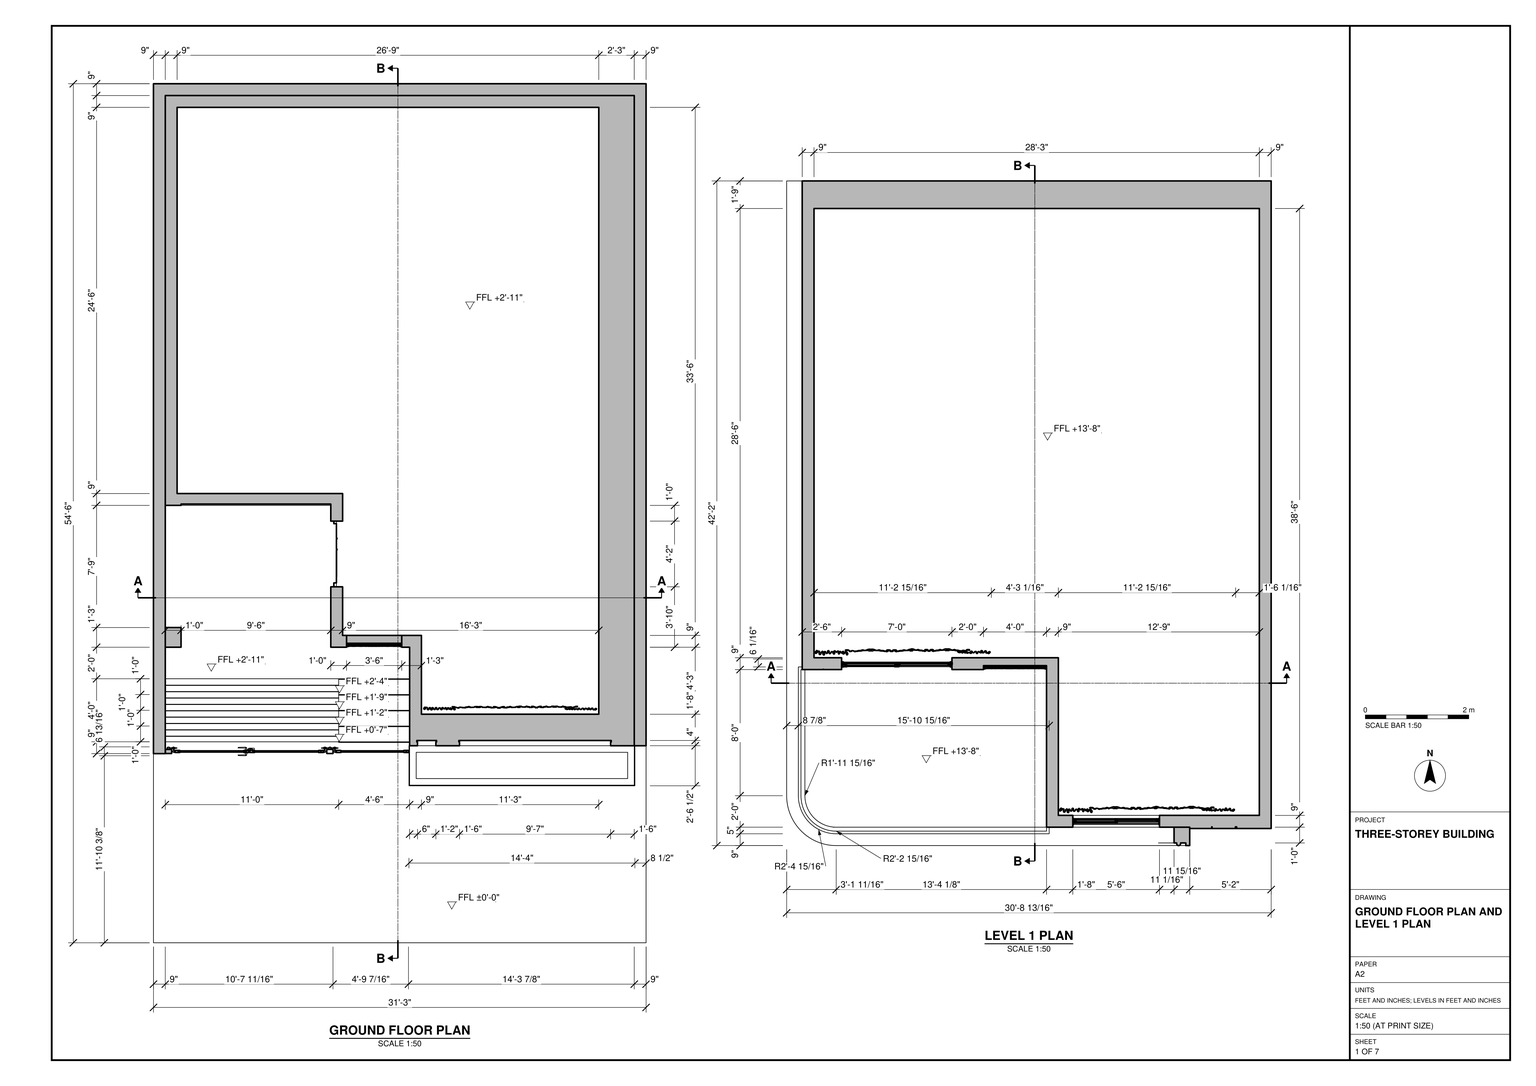
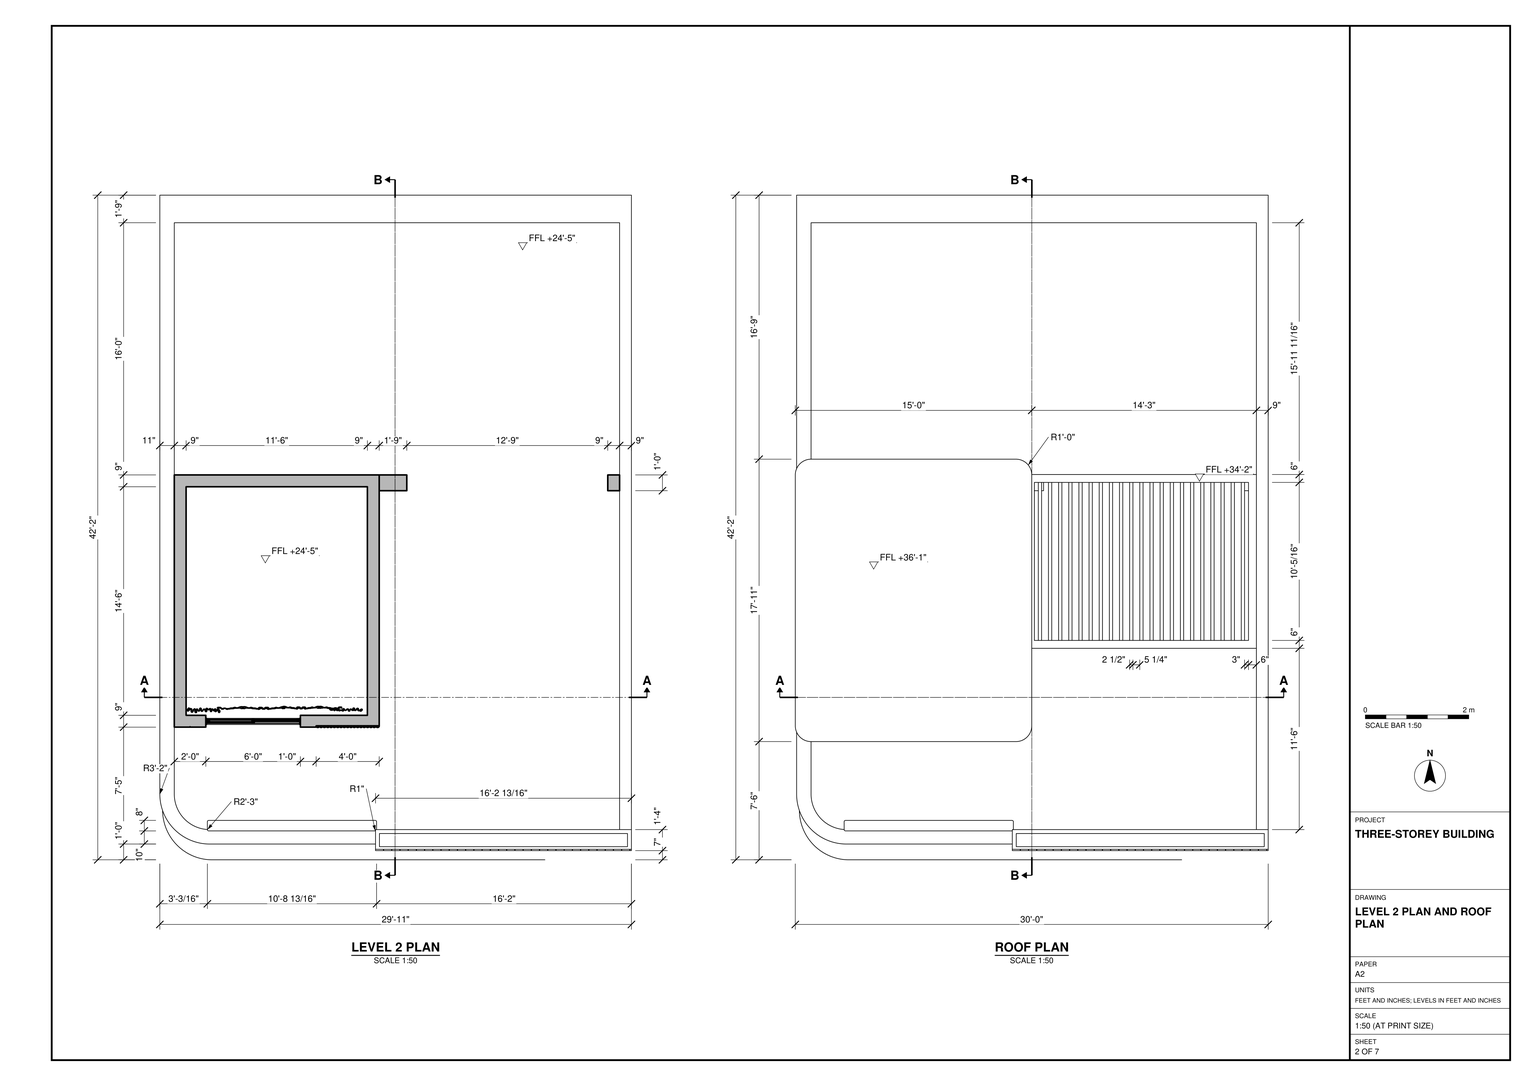
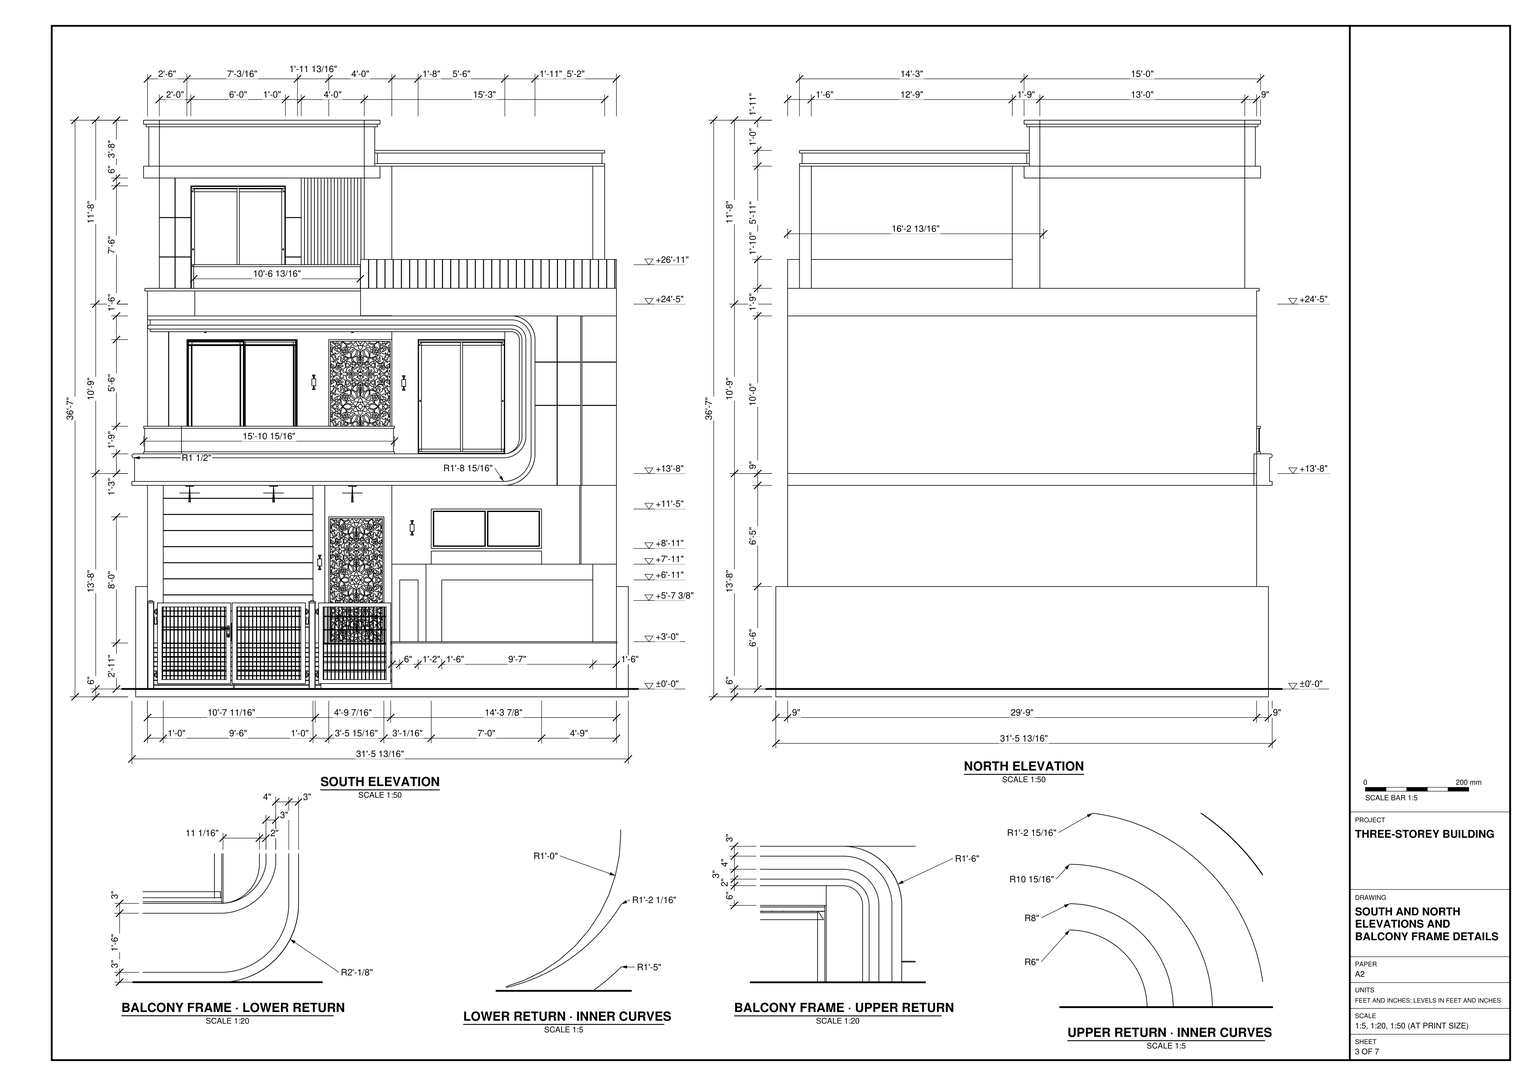
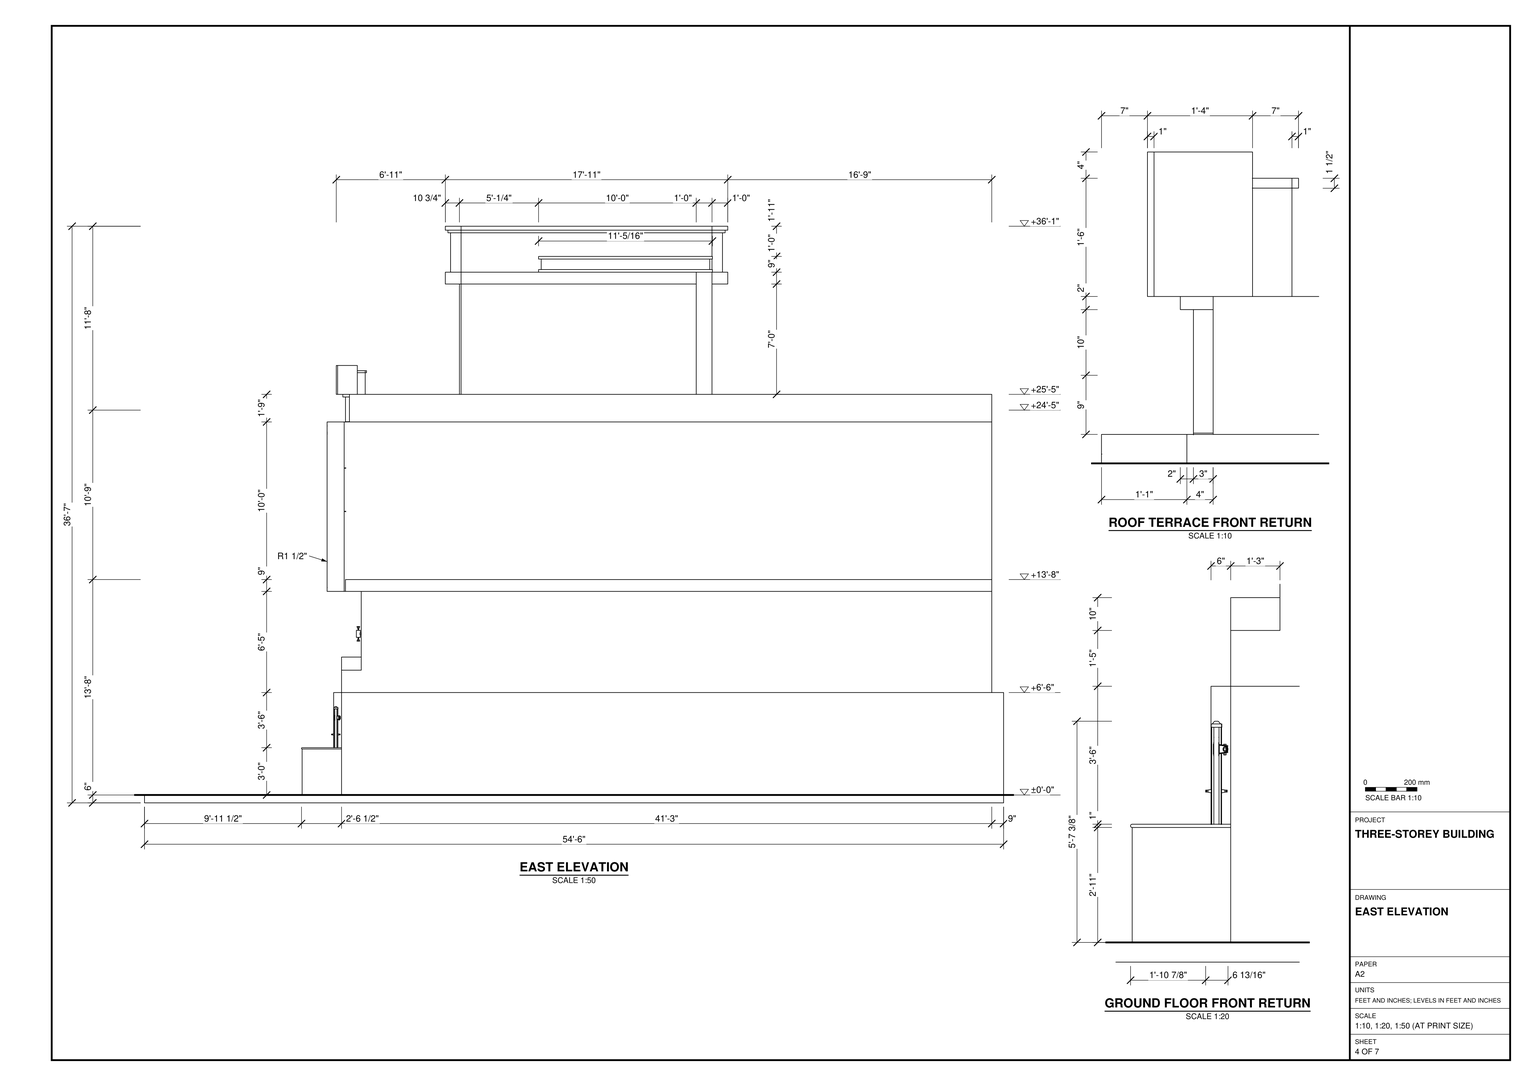
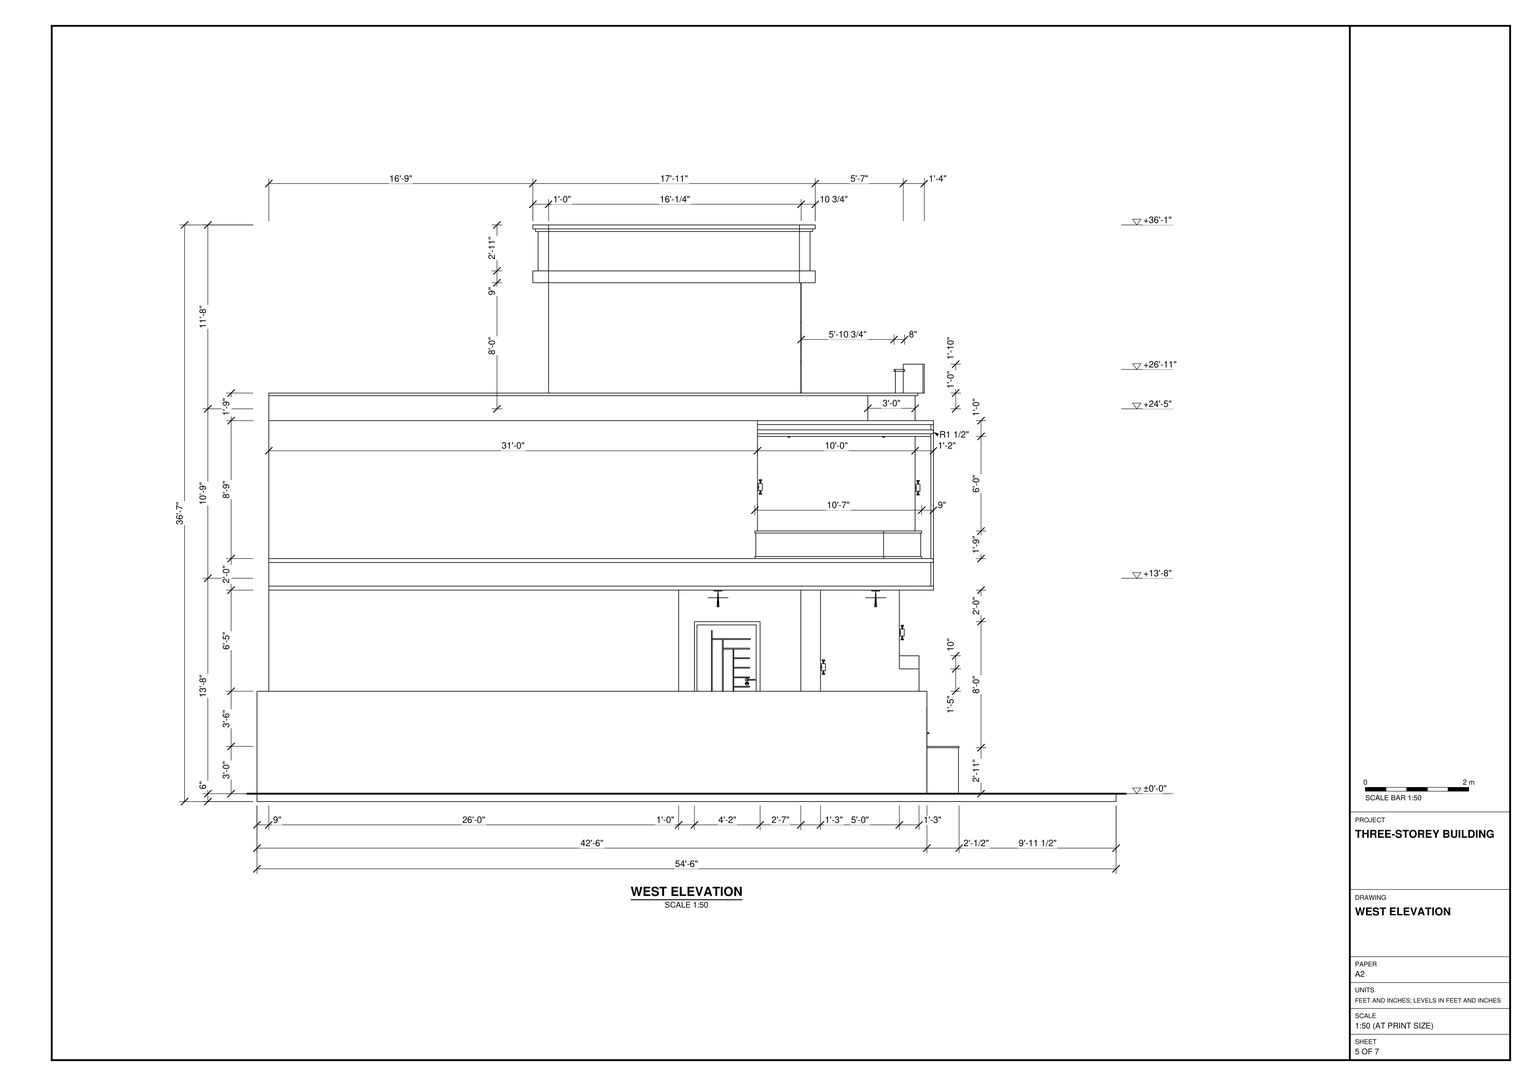
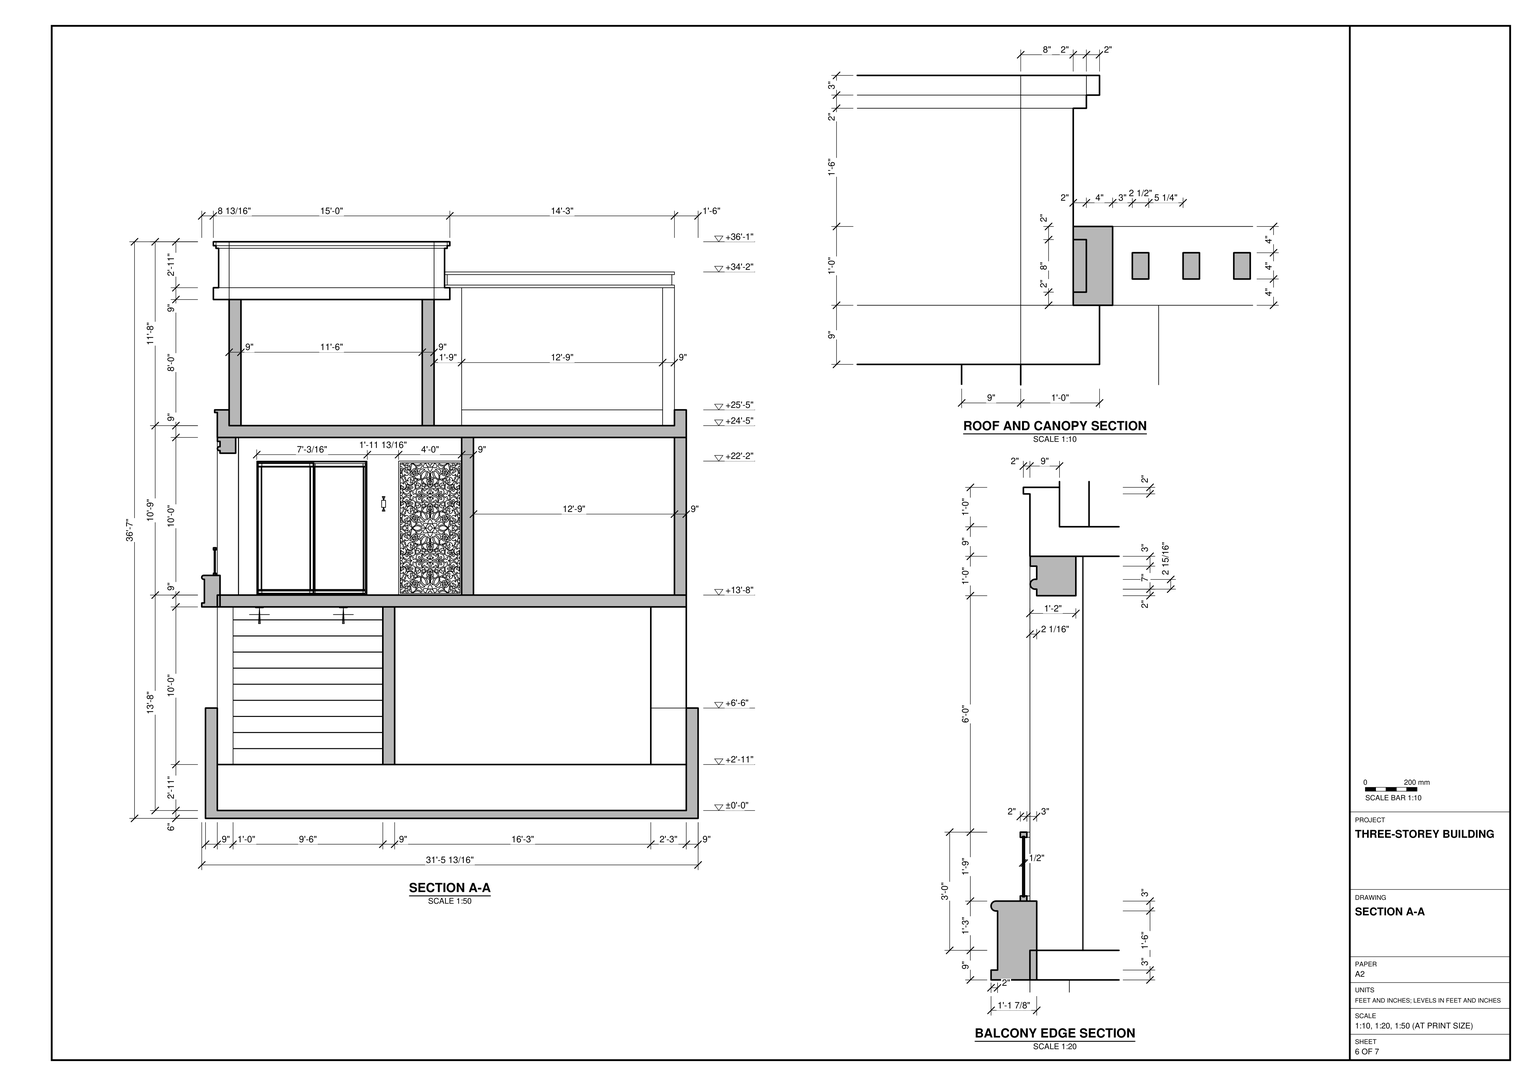
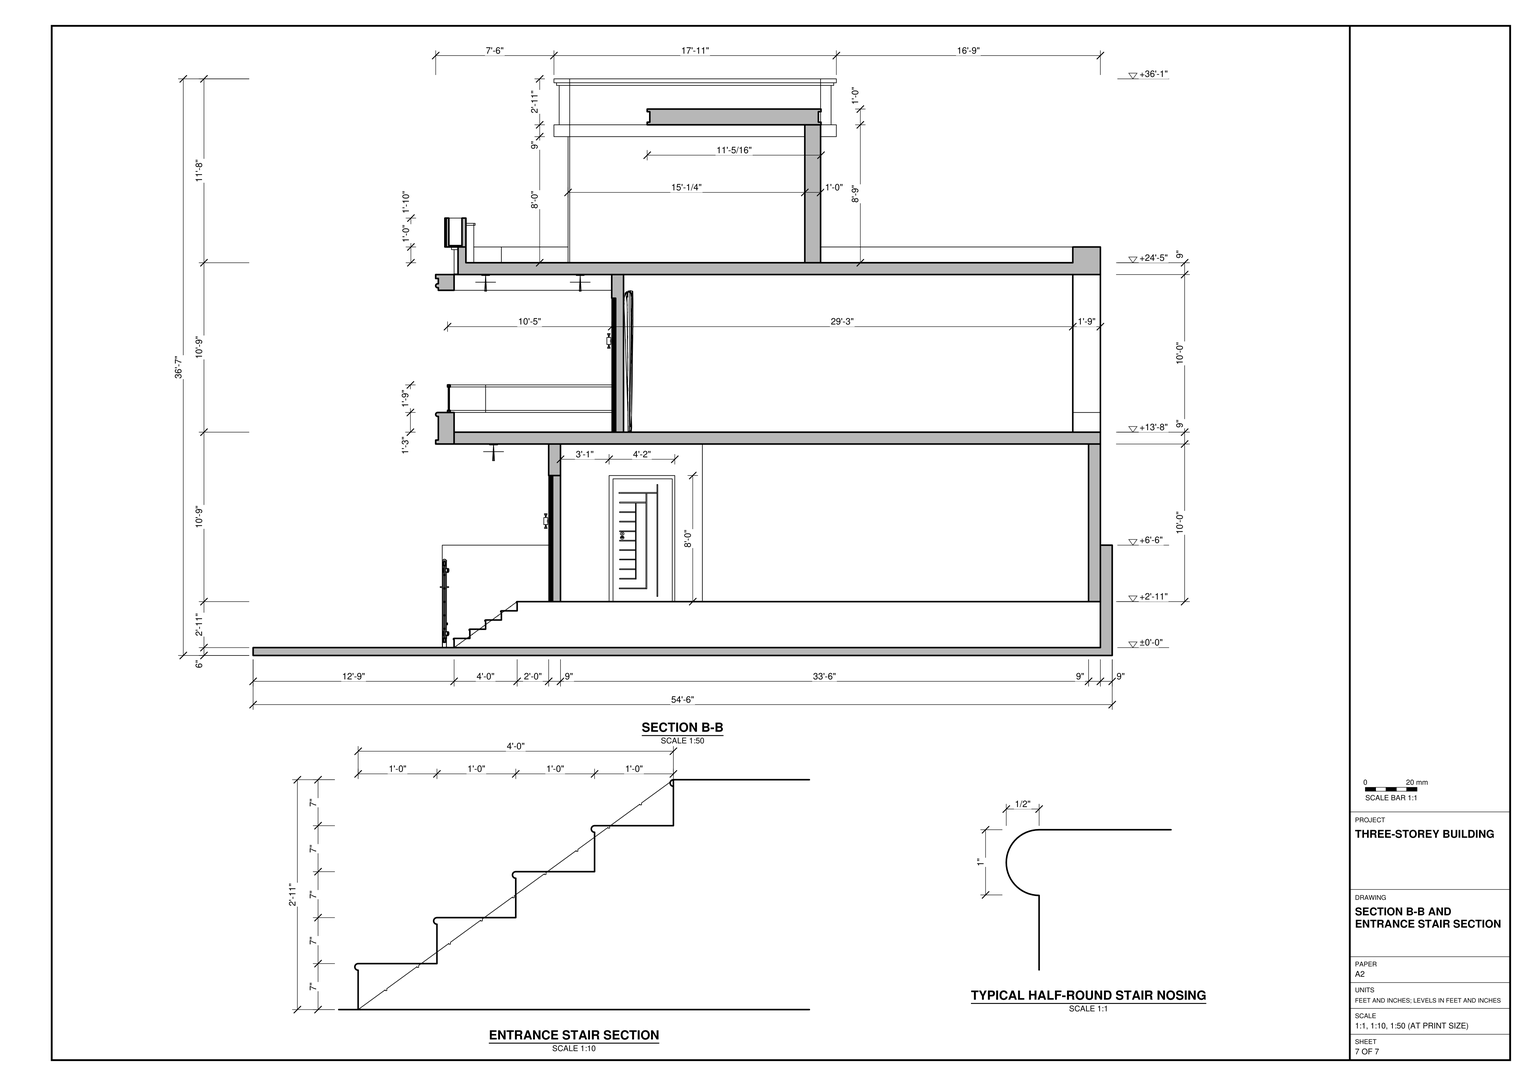
Build the three-storey building in SketchUp from task_files/diagram_01.pdf. Work in feet and inches. The complete model is 31'-5 13/16" wide along X, 54'-6" deep along Y and 36'-7" high along Z. Set out the storey levels at ±0'-0", +13'-8" and +24'-5". Distinguish the ground datum from the raised entrance floor at +2'-11".

Use the plans to lay out the forecourt, entrance steps, walls, floor slabs and openings. Follow the wall thicknesses and changes in footprint shown on each floor. On the south elevation, model the entrance gates, screen panels and framed glazing. At level 1, set the left opening back behind the balcony and carry the layered horizontal frame around the right opening, using the enlarged details for its curved returns. At level 2, place the smaller enclosed room to the left of the open terrace. Include the terrace edge, the flat roof over the room and the adjoining slatted canopy.

Keep walls, slabs and roof elements in separate groups or components. Group each furniture or built-in joinery piece shown separately, and use components for repeated parts. Decor and loose items may be any suitable library components, for example from 3D Warehouse. Save one SketchUp model as output_files/three_storey_building_with_a_curved_balcony_frame.skp.

# SketchUp Ruby script. Lengths in inches.
U = 1.inch
M = Sketchup.active_model
def pt(a) = Geom::Point3d.new(a.map { |v| v * U })
def face(e, loops, mat)
  f = e.add_face(loops[0].map { |a| pt(a) })
  loops[1..].each { |l| e.add_face(l.map { |a| pt(a) }).erase! }
  f.material = f.back_material = mat if mat
  f
end
# faces: each face lists its corners as indices into pts; further lists are holes
def faces(e, pts, list, mat = nil) = list.each { |f| face(e, (f[0].is_a?(Array) ? f : [f]).map { |l| l.map { |i| pts[i] } }, mat) }
# xy, xz, yz: faces in a plane at the given z, y or x. An outline is a flat list of corners, or four numbers for a rectangle; further outlines are holes
def ring(l) = l.size == 4 ? [[l[0], l[1]], [l[2], l[1]], [l[2], l[3]], [l[0], l[3]]] : l.each_slice(2).to_a
def flat(e, list, mat, &to3) = list.each { |f| face(e, (f[0].is_a?(Array) ? f : [f]).map { |l| ring(l).map { |u, v| to3.(u, v) } }, mat) }
def xy(e, z, list, mat = nil) = flat(e, list, mat) { |x, y| [x, y, z] }
def xz(e, y, list, mat = nil) = flat(e, list, mat) { |x, z| [x, y, z] }
def yz(e, x, list, mat = nil) = flat(e, list, mat) { |y, z| [x, y, z] }
def lines(e, pts, list) = list.each { |a, b| e.add_line(pt(pts[a]), pt(pts[b])) }
# prism: a flat outline (further loops are holes) pulled along v
def prism(e, loops, v, mat = nil)
  f = face(e, loops, mat); d = Geom::Vector3d.new(v.map { |x| x * U })
  f.pushpull(f.normal.samedirection?(d) ? d.length : -d.length)
end
def box(e, o, s, mat = nil) = prism(e, [[o, [o[0] + s[0], o[1], o[2]], [o[0] + s[0], o[1] + s[1], o[2]], [o[0], o[1] + s[1], o[2]]]], [0, 0, s[2]], mat)
def at(x, y, z, deg = 0) = Geom::Transformation.translation(pt([x, y, z])) * Geom::Transformation.rotation(ORIGIN, Z_AXIS, deg.degrees)
def axes(o, x, y, z) = Geom::Transformation.new([*x, 0, *y, 0, *z, 0, *pt(o).to_a, 1])
def part(name) = M.definitions.add(name)
# library, detail: a bought-in or finely detailed component or shape, given as its bounding box
def library(name, o, s) = part(name).tap { |d| box(d.entities, o, s) }
def detail(e, o, s) = box(e.add_group.entities, o, s)
def put(e, d, t, mat = nil) = e.add_instance(d, t).tap { |i| i.material = mat if mat }
def group(e, t, mat = nil) = e.add_group.tap { |g| g.transformation = t; g.material = mat if mat }.entities
root = M.entities
M.materials.add("1512 AP 8301 COAL MINE").color = [80, 80, 77]
M.materials.add("2020-01-14").color = [62, 53, 52]
M.materials.add("Wall Light").color = [248, 213, 137]
M.materials.add("[0136_Charcoal]").color = [35, 35, 35]
M.materials.add("[Color A05]").color = [255, 0, 0]
M.materials.add("[Formica Beige]").color = [235, 120, 86]
M.materials.add("[Formica Graystone]").color = [224, 223, 219]
M.materials.add("[Granite Tile]").color = [182, 180, 179]
M.materials.add("[Metal Corrugated Shiny]").color = [193, 193, 193]
M.materials.add("[Metal Rusted]").color = [135, 86, 63]
M.materials.add("[Stone Flagstone Ashlar]").color = [109, 109, 109]
M.materials.add("[Translucent Glass Blue]").color = [177, 191, 215]
M.materials.add("[Translucent Glass Blue]1").color = [190, 201, 222]
M.materials.add("[Wood Cherry Original]").color = [134, 83, 48]
M.materials.add("[Wood Veneer 01]").color = [96, 60, 36]
c1 = library("Lattice screen panel",[0,0,-3],[165.74,168.8125,3])
c2 = part("Decorative lattice screen")
put(c2.entities,c1,at(0,0,3))
put(c2.entities,c1,axes([0,675.25,3],[1,0,0],[0,-1,0],[0,0,1]))
put(c2.entities,c1,axes([331.47,0,3],[-1,0,0],[0,1,0],[0,0,1]))
put(c2.entities,c1,at(331.47,675.25,3,180))
put(c2.entities,c1,at(331.47,337.625,3,180))
put(c2.entities,c1,at(0,337.625,3))
put(c2.entities,c1,axes([331.47,337.625,3],[-1,0,0],[0,1,0],[0,0,1]))
put(c2.entities,c1,axes([0,337.625,3],[1,0,0],[0,-1,0],[0,0,1]))
c3 = part("Jali")
put(c3.entities,c2,at(55.22,75.56,-3),"[Metal Rusted]")
g1 = group(c3.entities,at(46.22,66.56,-6))
prism(g1,[[[0,0,0],[0,693.25,0],[349.47,693.25,0],[349.47,0,0]],[[340.47,9,0],[340.47,684.25,0],[9,684.25,0],[9,9,0]]],[0,0,9])
g2 = group(c3.entities,at(46.22,66.56,-15))
g3 = group(g2,at(0,0,0))
prism(g3,[[[0,0,0],[0,693.25,0],[349.47,693.25,0],[349.47,0,0]],[[340.47,9,0],[340.47,684.25,0],[9,684.25,0],[9,9,0]]],[0,0,9])
g4 = group(g2,at(9,9,2.08))
box(g4,[0,0,0],[331.47,675.25,3.9375],"[Translucent Glass Blue]1")
c4 = library("Metal mesh gate",[0,-1.63,0],[123.41,6.81,51.8125])
c5 = library("Component_63",[0,-41.05,1.35],[7.23,156.73,136.43])
c6 = library("WALL LIGHT 69",[4.19,4.05,-8.78],[4.61,5.7,17.13])
c7 = library("Group\#6",[-18,-30.5,-36],[357.5,525.5,36])
c8 = part("Door lever handle")
xz(c8.entities,1.97,[[0.3,0,0.15,0.04,0.04,0.15,0,0.3,0.04,0.44,0.15,0.55,0.3,0.59,0.44,0.55,0.55,0.44,0.59,0.3,0.55,0.15,0.44,0.04]])
yz(c8.entities,4.72,[[0.3,0,0.44,0.04,0.55,0.15,0.59,0.3,0.55,0.44,0.44,0.55,0.3,0.59,0.15,0.55,0.04,0.44,0,0.3,0.04,0.15,0.15,0.04]],"[Metal Corrugated Shiny]")
p = [[0.04,1.97,0.15],[0.15,1.97,0.04],[0.15,0.15,0.04],[0.04,0.04,0.15],[4.72,0.15,0.04],[4.72,0.04,0.15],
  [0.3,1.97,0],[0.3,0.3,0],[4.72,0.3,0],[0.44,1.97,0.04],[0.44,0.44,0.04],[4.72,0.44,0.04],
  [0.55,1.97,0.15],[0.55,0.55,0.15],[4.72,0.55,0.15],[0,1.97,0.3],[0,0,0.3],[4.72,0,0.3],
  [0.59,1.97,0.3],[0.59,0.59,0.3],[4.72,0.59,0.3],[0.04,1.97,0.44],[0.04,0.04,0.44],[4.72,0.04,0.44],
  [0.55,1.97,0.44],[0.55,0.55,0.44],[4.72,0.55,0.44],[0.15,1.97,0.55],[0.15,0.15,0.55],[4.72,0.15,0.55],
  [0.44,1.97,0.55],[0.44,0.44,0.55],[4.72,0.44,0.55],[0.3,1.97,0.59],[0.3,0.3,0.59],[4.72,0.3,0.59]]
faces(c8.entities,p,[[0,1,2,3],[3,2,4,5],[1,6,7,2],[2,7,8,4],[6,9,10,7],[7,10,11,8],[9,12,13,10],[10,13,14,11],
  [15,0,3,16],[16,3,5,17],[12,18,19,13],[13,19,20,14],[21,15,16,22],[22,16,17,23],[18,24,25,19],[19,25,26,20],
  [27,21,22,28],[28,22,23,29],[24,30,31,25],[25,31,32,26],[33,27,28,34],[34,28,29,35],[30,33,34,31],[31,34,35,32]],"[Metal Corrugated Shiny]")
c9 = part("Door handle rose")
xy(c9.entities,0,[[0.72,0,1.25,0.31]],"[Metal Corrugated Shiny]")
xy(c9.entities,1.97,[[0.72,0,1.25,0.31]],"[Metal Corrugated Shiny]")
xz(c9.entities,0,[[0.72,0,1.25,0,1.71,0.26,1.97,0.72,1.97,1.25,1.71,1.71,1.25,1.97,0.72,1.97,0.26,1.71,0,1.25,0,0.72,0.26,0.26]],"[Metal Corrugated Shiny]")
yz(c9.entities,0,[[0,0.72,0.31,1.25]],"[Metal Corrugated Shiny]")
yz(c9.entities,1.97,[[0,0.72,0.31,1.25]],"[Metal Corrugated Shiny]")
p = [[0.26,0.31,0.26],[0.72,0.31,0],[0.72,0,0],[0.26,0,0.26],[1.25,0.31,0],[1.71,0.31,0.26],
  [1.71,0,0.26],[1.25,0,0],[0,0.31,0.72],[0,0,0.72],[1.97,0.31,0.72],[1.97,0,0.72],
  [0.26,0.31,1.71],[0,0.31,1.25],[0,0,1.25],[0.26,0,1.71],[1.97,0.31,1.25],[1.71,0.31,1.71],
  [1.71,0,1.71],[1.97,0,1.25],[0.72,0.31,1.97],[0.72,0,1.97],[1.25,0.31,1.97],[1.25,0,1.97]]
faces(c9.entities,p,[[0,1,2,3],[4,5,6,7],[8,0,3,9],[5,10,11,6],[12,13,14,15],[16,17,18,19],[20,12,15,21],[17,22,23,18]],"[Metal Corrugated Shiny]")
c10 = part("Flush door")
g5 = group(c10.entities,at(6.7,3.07,40.99))
g6 = group(g5,at(0,-2.36,-0.39))
xy(g6,0.39,[[-1.03,-0.31,-0.59,0]],"[Metal Corrugated Shiny]")
xy(g6,1.38,[[-1.42,-0.12,-1.26,0],[-0.37,-0.12,-0.2,0]],"[Metal Corrugated Shiny]")
xy(g6,2.36,[[-1.03,-0.31,-0.59,0]],"[Metal Corrugated Shiny]")
xz(g6,-0.2,[[-0.8125,1.08,-0.85,1.1,-0.85,1.66,-0.8125,1.67,-0.77,1.66,-0.77,1.1]],"[Metal Corrugated Shiny]")
xz(g6,-0.12,[[-1.42,1.38,-1.34,1.75,-1.12,2.02,-0.8125,2.12,-0.51,2.02,-0.28,1.75,-0.2,1.38,-0.37,1.38,-0.42,1.65,-0.59,1.85,-0.8125,1.92,-1.03,1.85,-1.2,1.65,-1.26,1.38]],"[Color A05]")
xz(g6,-0.12,[[-0.85,1.1,-0.93,1.12,-1.02,1.23,-1.05,1.38,-1.02,1.53,-0.93,1.63,-0.85,1.66],[-0.77,1.1,-0.77,1.66,-0.69,1.63,-0.6,1.53,-0.57,1.38,-0.6,1.23,-0.69,1.12]],"[Metal Corrugated Shiny]")
xz(g6,0,[[[-1.03,0.39,-1.41,0.66,-1.62,1.11,-1.62,1.64,-1.41,2.1,-1.03,2.36,-0.59,2.36,-0.22,2.1,0,1.64,0,1.11,-0.22,0.66,-0.59,0.39],[-1.42,1.38,-1.26,1.38,-1.2,1.65,-1.03,1.85,-0.8125,1.92,-0.59,1.85,-0.42,1.65,-0.37,1.38,-0.2,1.38,-0.28,1.75,-0.51,2.02,-0.8125,2.12,-1.12,2.02,-1.34,1.75],[-0.8125,1.08,-0.69,1.12,-0.6,1.23,-0.57,1.38,-0.6,1.53,-0.69,1.63,-0.8125,1.67,-0.93,1.63,-1.02,1.53,-1.05,1.38,-1.02,1.23,-0.93,1.12]]],"[Metal Corrugated Shiny]")
yz(g6,-1.62,[[-0.31,1.11,0,1.64]],"[Metal Corrugated Shiny]")
yz(g6,-0.85,[[-0.2,1.1,-0.12,1.66]],"[Metal Corrugated Shiny]")
yz(g6,-0.77,[[-0.2,1.1,-0.12,1.66]],"[Metal Corrugated Shiny]")
yz(g6,0,[[-0.31,1.11,0,1.64]],"[Metal Corrugated Shiny]")
p = [[-1.03,-0.31,0.39],[-1.41,-0.31,0.66],[-1.41,0,0.66],[-1.03,0,0.39],[-0.22,-0.31,0.66],[-0.59,-0.31,0.39],
  [-0.59,0,0.39],[-0.22,0,0.66],[-1.62,-0.31,1.11],[-1.62,0,1.11],[0,-0.31,1.11],[0,0,1.11],
  [-0.8125,0,1.08],[-0.93,0,1.12],[-0.93,-0.12,1.12],[-0.85,-0.12,1.1],[-0.85,-0.2,1.1],[-0.8125,-0.2,1.08],
  [-0.69,0,1.12],[-0.77,-0.2,1.1],[-0.77,-0.12,1.1],[-0.69,-0.12,1.12],[-1.02,0,1.23],[-1.02,-0.12,1.23],
  [-0.6,0,1.23],[-0.6,-0.12,1.23],[-1.05,0,1.38],[-1.05,-0.12,1.38],[-0.57,0,1.38],[-0.57,-0.12,1.38],
  [-1.42,0,1.38],[-1.34,0,1.75],[-1.34,-0.12,1.75],[-1.42,-0.12,1.38],[-1.2,0,1.65],[-1.26,0,1.38],
  [-1.26,-0.12,1.38],[-1.2,-0.12,1.65],[-1.02,0,1.53],[-1.02,-0.12,1.53],[-0.6,0,1.53],[-0.6,-0.12,1.53],
  [-0.37,0,1.38],[-0.42,0,1.65],[-0.42,-0.12,1.65],[-0.37,-0.12,1.38],[-0.28,0,1.75],[-0.2,0,1.38],
  [-0.2,-0.12,1.38],[-0.28,-0.12,1.75],[-0.93,0,1.63],[-0.93,-0.12,1.63],[-0.69,0,1.63],[-0.69,-0.12,1.63],
  [-1.62,-0.31,1.64],[-1.41,-0.31,2.1],[-1.41,0,2.1],[-1.62,0,1.64],[-0.22,-0.31,2.1],[0,-0.31,1.64],
  [0,0,1.64],[-0.22,0,2.1],[-0.8125,0,1.67],[-0.8125,-0.2,1.67],[-0.85,-0.2,1.66],[-0.85,-0.12,1.66],
  [-0.77,-0.12,1.66],[-0.77,-0.2,1.66],[-1.03,0,1.85],[-1.03,-0.12,1.85],[-0.59,0,1.85],[-0.59,-0.12,1.85],
  [-1.12,0,2.02],[-1.12,-0.12,2.02],[-0.51,0,2.02],[-0.51,-0.12,2.02],[-0.8125,0,1.92],[-0.8125,-0.12,1.92],
  [-0.8125,0,2.12],[-0.8125,-0.12,2.12],[-1.03,-0.31,2.36],[-1.03,0,2.36],[-0.59,-0.31,2.36],[-0.59,0,2.36]]
faces(g6,p,[[0,1,2,3],[4,5,6,7],[1,8,9,2],[10,4,7,11],[12,13,14,15,16,17],[18,12,17,19,20,21],[13,22,23,14],[24,18,21,25],
  [22,26,27,23],[28,24,25,29],[30,31,32,33],[34,35,36,37],[26,38,39,27],[40,28,29,41],[42,43,44,45],[46,47,48,49],
  [38,50,51,39],[52,40,41,53],[54,55,56,57],[58,59,60,61],[50,62,63,64,65,51],[62,52,53,66,67,63],[68,34,37,69],[43,70,71,44],
  [31,72,73,32],[74,46,49,75],[76,68,69,77],[70,76,77,71],[72,78,79,73],[78,74,75,79],[55,80,81,56],[82,58,61,83]],"[Metal Corrugated Shiny]")
g7 = group(g5,at(0,0,0))
put(g7,c8,axes([-0.57,-0.39,3.25],[-0.82418,0,0],[0,-1,0],[0,0,1]))
put(g7,c9,axes([0,-2.36,2.56],[-0.82296,0,0],[0,-1,0],[0,0,0.99853]),"[Metal Corrugated Shiny]")
g8 = group(c10.entities,at(0,0.39,0))
xy(g8,0,[[0,0,1.76,1.97],[28.4,0,29.53,1.97]],"2020-01-14")
xy(g8,3.37,[[21.5,-0.39,21.89,0]],"2020-01-14")
xy(g8,8.39,[[4.57,-0.39,16.54,0],[16.54,-0.39,16.99,0]],"2020-01-14")
xy(g8,8.94,[[4.57,-0.39,16.54,0]],"2020-01-14")
xy(g8,14.74,[[4.72,-0.39,11.85,0],[11.85,-0.39,12.18,0]],"2020-01-14")
xy(g8,15.29,[[4.72,-0.39,11.85,0]],"2020-01-14")
xy(g8,20.96,[[4.72,-0.39,11.85,0]],"2020-01-14")
xy(g8,21.52,[[4.72,-0.39,11.85,0]],"2020-01-14")
xy(g8,27.37,[[4.72,-0.39,11.85,0]],"2020-01-14")
xy(g8,27.88,[[4.72,-0.39,11.85,0]],"2020-01-14")
xy(g8,33.55,[[4.72,-0.39,11.85,0]],"2020-01-14")
xy(g8,34.08,[[4.72,-0.39,11.85,0]],"2020-01-14")
xy(g8,39.69,[[4.72,-0.39,11.85,0]],"2020-01-14")
xy(g8,40.25,[[4.72,-0.39,11.85,0]],"2020-01-14")
xy(g8,45.86,[[4.72,-0.39,11.85,0]],"2020-01-14")
xy(g8,46.4,[[4.72,-0.39,11.85,0]],"2020-01-14")
xy(g8,52.16,[[4.72,-0.39,11.85,0]],"2020-01-14")
xy(g8,52.75,[[4.72,-0.39,11.85,0]],"2020-01-14")
xy(g8,58.4,[[4.72,-0.39,11.85,0]],"2020-01-14")
xy(g8,58.97,[[4.72,-0.39,11.85,0]],"2020-01-14")
xy(g8,64.58,[[4.72,-0.39,11.85,0],[12.18,-0.39,16.54,0]],"2020-01-14")
xy(g8,65.29,[[4.72,-0.39,16.54,0]],"2020-01-14")
xy(g8,70.95,[[4.43,-0.39,16.54,0],[16.99,-0.39,21.5,0]],"2020-01-14")
xy(g8,71.58,[[4.43,-0.39,21.5,0]],"2020-01-14")
xy(g8,76.79,[[21.5,-0.39,21.89,0]],"2020-01-14")
xy(g8,80.51,[[1.76,0,28.4,1.97]],"2020-01-14")
xy(g8,82.68,[[0,0,29.53,1.97]],"2020-01-14")
xz(g8,-0.39,[[21.5,3.37,21.89,76.79],[4.57,8.39,16.54,8.94],[16.54,8.39,16.99,70.95],[4.72,14.74,11.85,15.29],[11.85,14.74,12.18,64.58],
  [4.72,20.96,11.85,21.52],[4.72,27.37,11.85,27.88],[4.72,33.55,11.85,34.08],[4.72,39.69,11.85,40.25],[4.72,45.86,11.85,46.4],
  [4.72,52.16,11.85,52.75],[4.72,58.4,11.85,58.97],[4.72,64.58,16.54,65.29],[4.43,70.95,21.5,71.58]],"2020-01-14")
xz(g8,0,[[[1.76,0,28.4,80.51],[21.5,3.37,21.5,70.95,16.99,70.95,16.99,8.39,4.57,8.39,4.57,8.94,16.54,8.94,16.54,64.58,12.18,64.58,12.18,14.74,4.72,14.74,4.72,15.29,11.85,15.29,11.85,20.96,4.72,20.96,4.72,21.52,11.85,21.52,11.85,27.37,4.72,27.37,4.72,27.88,11.85,27.88,11.85,33.55,4.72,33.55,4.72,34.08,11.85,34.08,11.85,39.69,4.72,39.69,4.72,40.25,11.85,40.25,11.85,45.86,4.72,45.86,4.72,46.4,11.85,46.4,11.85,52.16,4.72,52.16,4.72,52.75,11.85,52.75,11.85,58.4,4.72,58.4,4.72,58.97,11.85,58.97,11.85,64.58,4.72,64.58,4.72,65.29,16.54,65.29,16.54,70.95,4.43,70.95,4.43,71.58,21.5,71.58,21.5,76.79,21.89,76.79,21.89,3.37]]],"2020-01-14")
xz(g8,1.97,[[0,0,1.76,0,1.76,80.51,28.4,80.51,28.4,0,29.53,0,29.53,82.68,0,82.68]],"2020-01-14")
yz(g8,0,[[0,0,1.97,82.68]],"2020-01-14")
yz(g8,1.76,[[0,0,1.97,80.51]],"2020-01-14")
yz(g8,4.43,[[-0.39,70.95,0,71.58]],"2020-01-14")
yz(g8,4.57,[[-0.39,8.39,0,8.94]],"2020-01-14")
yz(g8,4.72,[[-0.39,14.74,0,15.29],[-0.39,20.96,0,21.52],[-0.39,27.37,0,27.88],[-0.39,33.55,0,34.08],[-0.39,39.69,0,40.25],
  [-0.39,45.86,0,46.4],[-0.39,52.16,0,52.75],[-0.39,58.4,0,58.97],[-0.39,64.58,0,65.29]],"2020-01-14")
yz(g8,11.85,[[-0.39,15.29,0,20.96],[-0.39,21.52,0,27.37],[-0.39,27.88,0,33.55],[-0.39,34.08,0,39.69],[-0.39,40.25,0,45.86],
  [-0.39,46.4,0,52.16],[-0.39,52.75,0,58.4],[-0.39,58.97,0,64.58]],"2020-01-14")
yz(g8,12.18,[[-0.39,14.74,0,64.58]],"2020-01-14")
yz(g8,16.54,[[-0.39,8.94,0,64.58],[-0.39,65.29,0,70.95]],"2020-01-14")
yz(g8,16.99,[[-0.39,8.39,0,70.95]],"2020-01-14")
yz(g8,21.5,[[-0.39,3.37,0,70.95],[-0.39,71.58,0,76.79]],"2020-01-14")
yz(g8,21.89,[[-0.39,3.37,0,76.79]],"2020-01-14")
yz(g8,28.4,[[0,0,1.97,80.51]],"2020-01-14")
yz(g8,29.53,[[0,0,1.97,82.68]],"2020-01-14")
c11 = part("1")
prism(c11.entities,[[[39.75,0,0],[0,0,0],[0,0,27],[39.75,0,27]],[[0.5,0,0.5],[39.25,0,0.5],[39.25,0,26.5],[0.5,0,26.5]]],[0,-1,0])
g9 = group(c11.entities,at(0.5,-0.75,0.5),"[Translucent Glass Blue]")
box(g9,[0,0,0],[38.75,0.47,26])
c12 = part("Group5\#1")
box(c12.entities,[-48,-60,0],[96,12,1])
c13 = part("Group6\#1")
box(c13.entities,[-48,-47.75,0],[96,12,1])
c14 = part("Group7\#1")
box(c14.entities,[-48,-35.5,0],[96,12,1])
c15 = part("Group8\#1")
box(c15.entities,[-48,-23.25,0],[96,12,1])
c16 = part("Group9\#1")
box(c16.entities,[-48,-11,0],[96,12,1])
c17 = part("Group10\#1")
box(c17.entities,[-48,1.25,0],[96,12,1])
c18 = part("Group11\#1")
box(c18.entities,[-48,13.5,0],[96,12,1])
c19 = part("Group12\#1")
box(c19.entities,[-48,25.75,0],[96,12,1])
c20 = part("Group13\#1")
box(c20.entities,[-48,38,0],[96,12,1])
c21 = part("Group14\#1")
box(c21.entities,[-48,50.25,0],[96,9.75,1])
c22 = part("Group3\#1")
put(c22.entities,c12,at(0,0,0))
put(c22.entities,c13,at(0,0,0))
put(c22.entities,c14,at(0,0,0))
put(c22.entities,c15,at(0,0,0))
put(c22.entities,c16,at(0,0,0))
put(c22.entities,c17,at(0,0,0))
put(c22.entities,c18,at(0,0,0))
put(c22.entities,c19,at(0,0,0))
put(c22.entities,c20,at(0,0,0))
put(c22.entities,c21,at(0,0,0))
c23 = library("Group\#9",[-11.84,-14,-12.71],[368.84,506,141.71])
c24 = library("Group\#11",[-2.93,-5,-9],[359.93,497,129.2])
c25 = library("Group\#13",[-2,-7,-12.71],[359,499,55.71])
c26 = library("Group\#16",[0,-0.25,0],[156,192.25,96])
c27 = library("Group\#18",[-12,-12,0],[180,215,44])
c28 = part("3")
box(c28.entities,[1,-120.3125,0],[2.5,120.3125,4])
c29 = library("Group\#60",[0,0,0],[55.78,24.12,15.21])
g10 = group(root,at(27,165,30.82))
put(g10,c3,axes([114.45,60.86,-10.22],[0.12,0,0],[0,0,0.13848],[0,-0.12,0]),"[Wood Veneer 01]")
put(g10,c4,axes([-18,-21,-36],[1.5,0,0],[0,1,0],[0,0,1.3]))
put(g10,c5,axes([276.64,-3,236.85],[0,1,0],[-0.86133,0,0],[0,0,-0.79]))
put(g10,c5,axes([90.64,117,236.85],[0,1,0],[-0.86133,0,0],[0,0,-0.79]))
put(g10,c5,axes([99.64,84,365.85],[0,1,0],[-0.86133,0,0],[0,0,-0.79]))
put(g10,c6,axes([108.875,53.66,60.48],[0.65,0,0],[0,0.65,0],[0,0,0.65]))
put(g10,c6,axes([104.375,101.66,197.6],[0.65,0,0],[0,0.65,0],[0,0,0.65]))
put(g10,c6,axes([172.84,-18.34,197.08],[0.65,0,0],[0,0.65,0],[0,0,0.65]))
put(g10,c6,axes([179.21,-6.34,86.83],[0.65,0,0],[0,0.65,0],[0,0,0.65]))
put(g10,c7,at(0,-15,0),"[Formica Graystone]")
g11 = group(g10,at(-18,-15,-1))
xy(g11,0,[[186,0,186,75,180,75,180,84,195,84,195,24,330,24,330,486,9,486,9,192,135,192,135,171,126,171,126,184,12,184,12,183,0,183,0,495,357,495,357,0,339,0,339,3,339.5,3,339.5,4,223.5,4,223.5,3,224,3,224,0,206,0,206,3,206.5,3,206.5,4,191.5,4,191.5,3,192,3,192,0],[0,75,12,90],[126,75,126,121,135,121,135,84,138,84,138,75],[138,78,180,84]])
xy(g11,0.15,[[191.65,2.75,191.85,3],[206.15,2.75,206.35,3]])
xy(g11,0.16,[[223.66,2.75,223.84,3],[339.16,2.75,339.34,3]])
xy(g11,48,[[192,0,206,3]],"[Formica Beige]")
xy(g11,48,[[224,0,339,3]],"[Formica Graystone]")
xy(g11,48.15,[[191.85,2.75,206.15,3]])
xy(g11,48.16,[[223.84,2.75,339.16,3]])
xy(g11,48.34,[[223.66,2.75,339.34,3]])
xy(g11,48.35,[[191.65,2.75,206.35,3]])
xy(g11,48.5,[[223.5,3,339.5,4]])
xy(g11,48.5,[[191.5,3,206.5,4]],"[Formica Beige]")
xy(g11,60,[[186,0,357,0,357,15,330,15,330,15.5,329,15.5,329,15,186,15]])
xy(g11,72,[[216,15,300,24]])
xy(g11,96,[[138,75,180,78],[138,78,180,84]])
xy(g11,96,[[126,121,135,171]],"[Formica Graystone]")
xy(g11,102,[[216,15,300,24]])
xy(g11,120,[[[186,15,329,15,329,15.5,330,15.5,330,15,357,15,357,495,0,495,0,183,12,183,12,184,126,184,126,75,186,75],[195,24,195,84,135,84,135,192,9,192,9,486,330,486,330,24]],[0,75,12,90]])
xz(g11,0,[[186,0,192,0,192,48,206,48,206,0,212,0,212,60,186,60],[339,0,357,60]],"[Formica Beige]")
xz(g11,0,[[212,0,224,0,224,48,339,48,339,60,212,60]],"[Formica Graystone]")
xz(g11,2.75,[[191.65,0.15,191.65,48.35,206.35,48.35,206.35,0.15,206.15,0.15,206.15,48.15,191.85,48.15,191.85,0.15],[223.66,0.16,223.66,48.34,339.34,48.34,339.34,0.16,339.16,0.16,339.16,48.16,223.84,48.16,223.84,0.16]])
xz(g11,3,[[[191.5,0,191.5,48.5,206.5,48.5,206.5,0,206,0,206,48,192,48,192,0],[191.65,0.15,191.85,0.15,191.85,48.15,206.15,48.15,206.15,0.15,206.35,0.15,206.35,48.35,191.65,48.35]],[[223.5,0,223.5,48.5,339.5,48.5,339.5,0,339,0,339,48,224,48,224,0],[223.66,0.16,223.84,0.16,223.84,48.16,339.16,48.16,339.16,0.16,339.34,0.16,339.34,48.34,223.66,48.34]]])
xz(g11,4,[[191.5,0,206.5,48.5]],"[Formica Beige]")
xz(g11,4,[[223.5,0,339.5,48.5]],"[Formica Graystone]")
xz(g11,15,[[[186,60,329,120],[216,72,300,102]],[330,60,357,120]],"[Stone Flagstone Ashlar]")
xz(g11,15.5,[[329,60,330,120]])
xz(g11,24,[[[195,0,330,120],[216,72,300,102]]])
xz(g11,75,[[0,0,12,120],[126,0,135,120]],"[Formica Graystone]")
xz(g11,75,[[135,0,138,0,138,96,180,96,180,0,186,0,186,120,135,120]],"[Wood Cherry Original]")
xz(g11,78,[[138,0,180,96]])
xz(g11,84,[[135,0,135,120,195,120,195,0,180,0,180,96,138,96,138,0],[138,0,180,96]])
xz(g11,90,[[0,0,12,120]])
xz(g11,121,[[126,0,135,96]])
xz(g11,171,[[126,0,135,96]],"[Formica Graystone]")
xz(g11,183,[[0,0,12,120]],"[Formica Graystone]")
xz(g11,184,[[12,0,126,120]])
xz(g11,192,[[9,0,135,120]])
xz(g11,486,[[9,0,330,120]])
xz(g11,495,[[0,0,357,120]])
yz(g11,0,[[75,0,90,120],[183,0,495,120]],"[Formica Graystone]")
yz(g11,9,[[192,0,486,120]])
yz(g11,12,[[183,0,184,120]])
yz(g11,12,[[75,0,90,120]],"[Formica Graystone]")
yz(g11,126,[[75,0,75,120,184,120,184,0,171,0,171,96,121,96,121,0]],"[Formica Graystone]")
yz(g11,135,[[84,0,121,0,121,96,171,96,171,0,192,0,192,120,84,120]])
yz(g11,138,[[75,0,78,96],[78,0,84,96]])
yz(g11,180,[[75,0,78,96],[78,0,84,96]])
yz(g11,186,[[0,0,0,60,15,60,15,120,75,120,75,0]],"[Stone Flagstone Ashlar]")
yz(g11,191.5,[[3,0,4,48.5]],"[Formica Beige]")
yz(g11,191.65,[[2.75,0.15,3,48.35]])
yz(g11,191.85,[[2.75,0.15,3,48.15]])
yz(g11,192,[[0,0,3,48]],"[Formica Beige]")
yz(g11,195,[[24,0,84,120]])
yz(g11,206,[[0,0,3,48]],"[Formica Beige]")
yz(g11,206.15,[[2.75,0.15,3,48.15]])
yz(g11,206.35,[[2.75,0.15,3,48.35]])
yz(g11,206.5,[[3,0,4,48.5]],"[Formica Beige]")
yz(g11,216,[[15,72,24,102]])
yz(g11,223.5,[[3,0,4,48.5]])
yz(g11,223.66,[[2.75,0.16,3,48.34]])
yz(g11,223.84,[[2.75,0.16,3,48.16]])
yz(g11,224,[[0,0,3,48]],"[Formica Graystone]")
yz(g11,300,[[15,72,24,102]])
yz(g11,329,[[15,60,15.5,120]])
yz(g11,330,[[24,0,486,120],[15,60,15.5,120]])
yz(g11,339,[[0,0,3,48]],"[Formica Graystone]")
yz(g11,339.16,[[2.75,0.16,3,48.16]])
yz(g11,339.34,[[2.75,0.16,3,48.34]])
yz(g11,339.5,[[3,0,4,48.5]])
yz(g11,357,[[0,0,495,0,495,120,15,120,15,60,0,60]])
put(g11,c10,axes([130.68,121,0],[0,1.69333,0],[-1,0,0],[0,0,1.16114]))
put(g11,c5,axes([294.64,24,108.85],[0,1,0],[-0.86133,0,0],[0,0,-0.79]))
g12 = group(g11,at(216,18,72),"[0136_Charcoal]")
prism(g12,[[[0,0,0],[0,0,30],[84,0,30],[84,0,0]],[[41.25,0,1.5],[41.25,0,28.5],[1.5,0,28.5],[1.5,0,1.5]],[[42.75,0,1.5],[82.5,0,1.5],[82.5,0,28.5],[42.75,0,28.5]]],[0,-2,0])
put(g12,c11,at(1.5,-0.5,1.5))
put(g12,c11,at(42.75,-0.5,1.5))
g13 = group(g11,at(12,184,0))
put(g13,c22,axes([57,0,60],[1.1875,0,0],[0,0,1],[0,-1,0]),"[Wood Cherry Original]")
g14 = group(g11,at(216,0,60),"[Stone Flagstone Ashlar]")
xy(g14,0,[[0,0,84,15]])
xy(g14,1,[[2.5,2.5,81.5,12.5]])
xy(g14,10,[[[0,0,84,15],[2.5,2.5,81.5,12.5]]])
xz(g14,0,[[0,0,84,10]])
xz(g14,2.5,[[2.5,1,81.5,10]])
xz(g14,12.5,[[2.5,1,81.5,10]])
xz(g14,15,[[0,0,84,10]])
yz(g14,0,[[0,0,15,10]])
yz(g14,2.5,[[2.5,1,12.5,10]])
yz(g14,81.5,[[2.5,1,12.5,10]])
yz(g14,84,[[0,0,15,10]])
g15 = group(g11,at(329,15.5,60),"Wall Light")
box(g15,[0,-0.5,0],[1,0.5,60])
g16 = group(g11,at(191.65,2.75,0.15),"Wall Light")
prism(g16,[[[14.5,0,0],[14.7,0,0],[14.7,0,48.2],[0,0,48.2],[0,0,0],[0.2,0,0],[0.2,0,48],[14.5,0,48]]],[0,0.25,0])
g17 = group(g11,at(223.66,2.75,0.16),"Wall Light")
prism(g17,[[[0.18,0,0],[0.18,0,48],[115.5,0,48],[115.5,0,0],[115.68,0,0],[115.68,0,48.18],[0,0,48.18],[0,0,0]]],[0,0.25,0])
put(g10,c23,at(-18,-12,119))
put(g10,c24,at(-18,-12,128))
put(g10,c25,at(-18,-12,248))
put(g10,c26,at(-9,75,257))
put(g10,c27,at(-9,76,353),"[Formica Graystone]")
g18 = group(g10,at(147,255,257),"1512 AP 8301 COAL MINE")
xy(g18,105,[[[7.99,-120,183,12.3125],[13.99,-114,177,6.3125]]])
xy(g18,107,[[[7.99,-120,183,12.3125],[9.99,-118,181,10.3125]]])
xy(g18,115,[[[7.99,-120,183,12.3125],[9.99,-118,181,10.3125]]])
xy(g18,117,[[[7.99,-120,183,12.3125],[13.99,-114,177,6.3125]]])
xz(g18,-120,[[7.99,105,183,107],[7.99,115,183,117]])
xz(g18,-118,[[9.99,107,181,115]])
xz(g18,-114,[[13.99,105,177,117]])
xz(g18,6.3125,[[13.99,105,177,117]])
xz(g18,10.3125,[[9.99,107,181,115]])
xz(g18,12.3125,[[7.99,105,183,107],[7.99,115,183,117]])
yz(g18,7.99,[[-120,105,12.3125,107],[-120,115,12.3125,117]])
yz(g18,9.99,[[-118,107,10.3125,115]])
yz(g18,13.99,[[-114,105,6.3125,117]])
yz(g18,177,[[-114,105,6.3125,117]])
yz(g18,181,[[-118,107,10.3125,115]])
yz(g18,183,[[-120,105,12.3125,107],[-120,115,12.3125,117]])
put(g18,c28,at(170.5,6.3125,109))
put(g18,c28,at(162.77,6.3125,109))
put(g18,c28,at(155.05,6.3125,109))
put(g18,c28,at(147.32,6.3125,109))
put(g18,c28,at(139.6,6.3125,109))
put(g18,c28,at(131.875,6.3125,109))
put(g18,c28,at(124.15,6.3125,109))
put(g18,c28,at(116.42,6.3125,109))
put(g18,c28,at(108.7,6.3125,109))
put(g18,c28,at(100.97,6.3125,109))
put(g18,c28,at(93.25,6.3125,109))
put(g18,c28,at(85.52,6.3125,109))
put(g18,c28,at(77.8,6.3125,109))
put(g18,c28,at(70.07,6.3125,109))
put(g18,c28,at(62.35,6.3125,109))
put(g18,c28,at(54.62,6.3125,109))
put(g18,c28,at(46.9,6.3125,109))
put(g18,c28,at(39.17,6.3125,109))
put(g18,c28,at(31.44,6.3125,109))
put(g18,c28,at(23.72,6.3125,109))
put(g18,c28,at(15.99,6.3125,109))
g19 = group(g18,at(162,0,0))
xy(g19,0,[[12,0,21,12]])
xy(g19,105,[[12,0,21,12]])
xz(g19,0,[[12,0,21,105]])
xz(g19,12,[[12,0,21,105]])
yz(g19,12,[[0,0,12,105]])
yz(g19,21,[[0,0,12,105]])
# 1 loose lines left out
g20 = group(g18,at(0,0,0))
prism(g20,[[[21,12,0],[0,12,0],[0,12,96],[12,12,96],[12,12,105],[21,12,105]]],[0,-12,0])
# 1 loose lines left out
g21 = group(g10,at(-18,-45,-36))
xy(g21,-6,[[-9,-120,366,534]])
xy(g21,0,[[-9,-120,366,-120,366,30,357,30,357,525,0,525,0,24,-9,24]],"[Granite Tile]")
xy(g21,78,[[-9,24,0,24,0,525,357,525,357,30,366,30,366,534,-9,534]],"[Formica Graystone]")
xz(g21,-120,[[-9,-6,366,0]])
xz(g21,24,[[-9,0,0,78]],"[Formica Graystone]")
xz(g21,30,[[357,0,366,78]],"[Formica Graystone]")
xz(g21,525,[[0,0,357,78]])
xz(g21,534,[[-9,-6,366,78]])
yz(g21,-9,[[-120,-6,-120,0,24,0,24,78,534,78,534,-6]])
yz(g21,0,[[24,0,525,78]],"[Formica Graystone]")
yz(g21,357,[[30,0,525,78]])
yz(g21,366,[[-120,-6,534,-6,534,78,30,78,30,0,-120,0]],"[Formica Graystone]")
put(g10,c29,axes([3.83,163.8125,-1],[0,-2.64,0],[3.036,0,0],[0,0,3.67488]))
